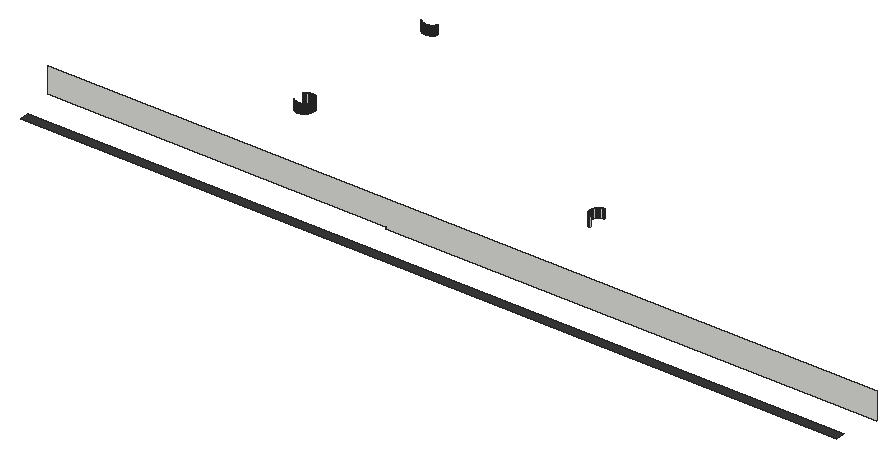
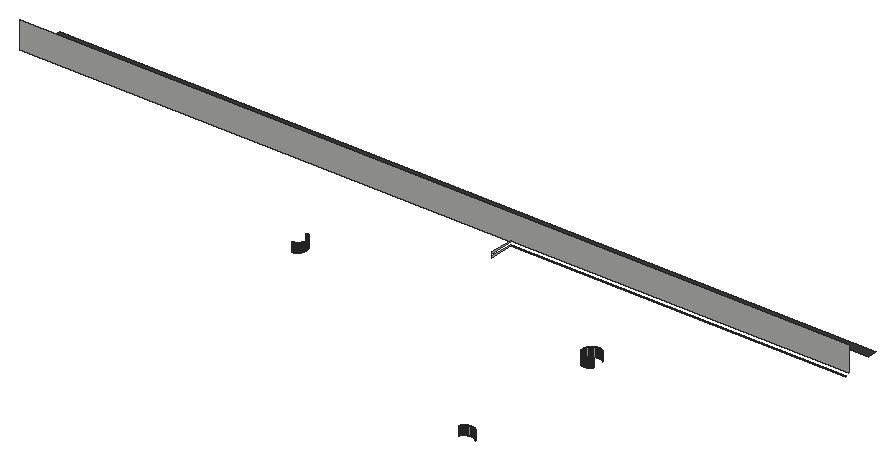
# SketchUp Ruby script. Lengths in inches.
U = 1.inch
M = Sketchup.active_model
def pt(a) = Geom::Point3d.new(a.map { |v| v * U })
def face(e, loops, mat)
  f = e.add_face(loops[0].map { |a| pt(a) })
  loops[1..].each { |l| e.add_face(l.map { |a| pt(a) }).erase! }
  f.material = f.back_material = mat if mat
  f
end
# faces: each face lists its corners as indices into pts; further lists are holes
def faces(e, pts, list, mat = nil) = list.each { |f| face(e, (f[0].is_a?(Array) ? f : [f]).map { |l| l.map { |i| pts[i] } }, mat) }
# xy, xz, yz: faces in a plane at the given z, y or x. An outline is a flat list of corners, or four numbers for a rectangle; further outlines are holes
def ring(l) = l.size == 4 ? [[l[0], l[1]], [l[2], l[1]], [l[2], l[3]], [l[0], l[3]]] : l.each_slice(2).to_a
def flat(e, list, mat, &to3) = list.each { |f| face(e, (f[0].is_a?(Array) ? f : [f]).map { |l| ring(l).map { |u, v| to3.(u, v) } }, mat) }
def xy(e, z, list, mat = nil) = flat(e, list, mat) { |x, y| [x, y, z] }
def xz(e, y, list, mat = nil) = flat(e, list, mat) { |x, z| [x, y, z] }
def yz(e, x, list, mat = nil) = flat(e, list, mat) { |y, z| [x, y, z] }
def lines(e, pts, list) = list.each { |a, b| e.add_line(pt(pts[a]), pt(pts[b])) }
# prism: a flat outline (further loops are holes) pulled along v
def prism(e, loops, v, mat = nil)
  f = face(e, loops, mat); d = Geom::Vector3d.new(v.map { |x| x * U })
  f.pushpull(f.normal.samedirection?(d) ? d.length : -d.length)
end
def box(e, o, s, mat = nil) = prism(e, [[o, [o[0] + s[0], o[1], o[2]], [o[0] + s[0], o[1] + s[1], o[2]], [o[0], o[1] + s[1], o[2]]]], [0, 0, s[2]], mat)
def at(x, y, z, deg = 0) = Geom::Transformation.translation(pt([x, y, z])) * Geom::Transformation.rotation(ORIGIN, Z_AXIS, deg.degrees)
def axes(o, x, y, z) = Geom::Transformation.new([*x, 0, *y, 0, *z, 0, *pt(o).to_a, 1])
def part(name) = M.definitions.add(name)
# library, detail: a bought-in or finely detailed component or shape, given as its bounding box
def library(name, o, s) = part(name).tap { |d| box(d.entities, o, s) }
def detail(e, o, s) = box(e.add_group.entities, o, s)
def put(e, d, t, mat = nil) = e.add_instance(d, t).tap { |i| i.material = mat if mat }
def group(e, t, mat = nil) = e.add_group.tap { |g| g.transformation = t; g.material = mat if mat }.entities
root = M.entities
M.materials.add("1496 AP 8293 CARBON COPY").color = [58, 58, 58]
xy(root,129,[[46,71,321,74]],"1496 AP 8293 CARBON COPY")
xz(root,85,[[158,129,323,129,323,138,44,138,44,129.5,158,129.5]])
xz(root,86.5,[[44,129,156.5,129.5]])
xz(root,119,[[100.84,129,100.92,132],[100.92,129,101,132],[101,129,101.08,132],[101.08,129,101.16,132]])
xz(root,125,[[100.84,129,100.92,132],[100.92,129,101,132],[101,129,101.08,132],[101.08,129,101.16,132]])
xz(root,172.75,[[100.84,129,100.92,132],[100.92,129,101,132],[101,129,101.08,132],[101.08,129,101.16,132]])
yz(root,104,[[121.84,129,121.92,132],[121.92,129,122,132],[122,129,122.08,132],[122.08,129,122.16,132]])
yz(root,156.5,[[86.5,129,94.5,129.5]])
yz(root,158,[[85,129,93,129.5]])
yz(root,197,[[121.84,129,121.92,132],[121.92,129,122,132],[122,129,122.08,132],[122.08,129,122.16,132]])
p = [[100.53,119.04,129],[100.45,119.05,129],[100.45,119.05,132],[100.53,119.04,132],[100.61,119.03,129],[100.61,119.03,132],
  [100.6875,119.02,129],[100.6875,119.02,132],[100.76,119.01,129],[100.76,119.01,132],[100.84,119,129],[100.84,119,132],
  [101.24,119.01,129],[101.16,119,129],[101.16,119,132],[101.24,119.01,132],[101.3125,119.02,129],[101.3125,119.02,132],
  [101.39,119.03,129],[101.39,119.03,132],[101.47,119.04,129],[101.47,119.04,132],[101.55,119.05,129],[101.55,119.05,132],
  [199.53,119.04,129],[199.45,119.05,129],[199.45,119.05,132],[199.53,119.04,132],[100.07,119.15,129],[100,119.17,129],
  [100,119.17,132],[100.07,119.15,132],[100.15,119.125,129],[100.15,119.125,132],[100.22,119.1,129],[100.22,119.1,132],
  [100.3,119.08,129],[100.3,119.08,132],[100.375,119.07,129],[100.375,119.07,132],[101.625,119.07,129],[101.625,119.07,132],
  [101.7,119.08,129],[101.7,119.08,132],[101.78,119.1,129],[101.78,119.1,132],[101.85,119.125,129],[101.85,119.125,132],
  [101.93,119.15,129],[101.93,119.15,132],[102,119.17,129],[102,119.17,132],[199.07,119.15,129],[199,119.17,129],
  [199,119.17,132],[199.07,119.15,132],[199.15,119.125,129],[199.15,119.125,132],[199.22,119.1,129],[199.22,119.1,132],
  [199.3,119.08,129],[199.3,119.08,132],[199.375,119.07,129],[199.375,119.07,132],[99.85,119.23,129],[99.78,119.26,129],
  [99.78,119.26,132],[99.85,119.23,132],[99.92,119.2,129],[99.92,119.2,132],[102.08,119.2,129],[102.08,119.2,132],
  [102.15,119.23,129],[102.15,119.23,132],[102.22,119.26,129],[102.22,119.26,132],[198.85,119.23,129],[198.78,119.26,129],
  [198.78,119.26,132],[198.85,119.23,132],[198.92,119.2,129],[198.92,119.2,132],[99.64,119.33,129],[99.57,119.36,129],
  [99.57,119.36,132],[99.64,119.33,132],[99.71,119.29,129],[99.71,119.29,132],[102.29,119.29,129],[102.29,119.29,132],
  [102.36,119.33,129],[102.36,119.33,132],[102.43,119.36,129],[102.43,119.36,132],[198.64,119.33,129],[198.57,119.36,129],
  [198.57,119.36,132],[198.64,119.33,132],[198.71,119.29,129],[198.71,119.29,132],[99.43,119.44,129],[99.37,119.48,129],
  [99.37,119.48,132],[99.43,119.44,132],[99.5,119.4,129],[99.5,119.4,132],[102.5,119.4,129],[102.5,119.4,132],
  [102.57,119.44,129],[102.57,119.44,132],[102.63,119.48,129],[102.63,119.48,132],[198.43,119.44,129],[198.37,119.48,129],
  [198.37,119.48,132],[198.43,119.44,132],[198.5,119.4,129],[198.5,119.4,132],[99.3,119.53,129],[99.24,119.57,129],
  [99.24,119.57,132],[99.3,119.53,132],[102.7,119.53,129],[102.7,119.53,132],[102.76,119.57,129],[102.76,119.57,132],
  [198.3,119.53,129],[198.24,119.57,129],[198.24,119.57,132],[198.3,119.53,132],[99.17,119.62,129],[99.11,119.67,129],
  [99.11,119.67,132],[99.17,119.62,132],[102.83,119.62,129],[102.83,119.62,132],[102.89,119.67,129],[102.89,119.67,132],
  [198.17,119.62,129],[198.11,119.67,129],[198.11,119.67,132],[198.17,119.62,132],[99.05,119.72,129],[98.99,119.77,129],
  [98.99,119.77,132],[99.05,119.72,132],[102.95,119.72,129],[102.95,119.72,132],[103.01,119.77,129],[103.01,119.77,132],
  [198.05,119.72,129],[197.99,119.77,129],[197.99,119.77,132],[198.05,119.72,132],[98.93,119.82,129],[98.88,119.88,129],
  [98.88,119.88,132],[98.93,119.82,132],[103.07,119.82,129],[103.07,119.82,132],[103.12,119.88,129],[103.12,119.88,132],
  [197.93,119.82,129],[197.88,119.88,129],[197.88,119.88,132],[197.93,119.82,132],[98.82,119.93,129],[98.77,119.99,129],
  [98.77,119.99,132],[98.82,119.93,132],[103.18,119.93,129],[103.18,119.93,132],[103.23,119.99,129],[103.23,119.99,132],
  [197.82,119.93,129],[197.77,119.99,129],[197.77,119.99,132],[197.82,119.93,132],[98.72,120.05,129],[98.72,120.05,132],
  [103.28,120.05,129],[103.28,120.05,132],[197.72,120.05,129],[197.72,120.05,132],[103.33,120.11,129],[103.33,120.11,132],
  [103.38,120.17,129],[103.38,120.17,132],[197.67,120.11,129],[197.62,120.17,129],[197.62,120.17,132],[197.67,120.11,132],
  [103.43,120.24,129],[103.43,120.24,132],[103.47,120.3,129],[103.47,120.3,132],[197.57,120.24,129],[197.53,120.3,129],
  [197.53,120.3,132],[197.57,120.24,132],[103.52,120.37,129],[103.52,120.37,132],[197.48,120.37,129],[197.48,120.37,132],
  [103.56,120.43,129],[103.56,120.43,132],[103.6,120.5,129],[103.6,120.5,132],[197.44,120.43,129],[197.4,120.5,129],
  [197.4,120.5,132],[197.44,120.43,132],[103.64,120.57,129],[103.64,120.57,132],[197.36,120.57,129],[197.36,120.57,132],
  [103.67,120.64,129],[103.67,120.64,132],[103.71,120.71,129],[103.71,120.71,132],[197.33,120.64,129],[197.29,120.71,129],
  [197.29,120.71,132],[197.33,120.64,132],[103.74,120.78,129],[103.74,120.78,132],[197.26,120.78,129],[197.26,120.78,132],
  [103.77,120.85,129],[103.77,120.85,132],[197.23,120.85,129],[197.23,120.85,132],[103.8,120.92,129],[103.8,120.92,132],
  [103.83,121,129],[103.83,121,132],[197.2,120.92,129],[197.17,121,129],[197.17,121,132],[197.2,120.92,132],
  [103.85,121.07,129],[103.85,121.07,132],[197.15,121.07,129],[197.15,121.07,132],[103.875,121.15,129],[103.875,121.15,132],
  [103.9,121.22,129],[103.9,121.22,132],[197.125,121.15,129],[197.1,121.22,129],[197.1,121.22,132],[197.125,121.15,132],
  [103.92,121.3,129],[103.92,121.3,132],[197.08,121.3,129],[197.08,121.3,132],[103.93,121.375,129],[103.93,121.375,132],
  [197.07,121.375,129],[197.07,121.375,132],[103.95,121.45,129],[103.95,121.45,132],[197.05,121.45,129],[197.05,121.45,132],
  [103.96,121.53,129],[103.96,121.53,132],[103.97,121.61,129],[103.97,121.61,132],[197.04,121.53,129],[197.03,121.61,129],
  [197.03,121.61,132],[197.04,121.53,132],[103.98,121.6875,129],[103.98,121.6875,132],[197.02,121.6875,129],[197.02,121.6875,132],
  [103.99,121.76,129],[103.99,121.76,132],[197.01,121.76,129],[197.01,121.76,132],[104,121.84,129],[104,121.84,132],
  [197,121.84,129],[197,121.84,132],[103.98,122.3125,129],[103.99,122.24,129],[103.99,122.24,132],[103.98,122.3125,132],
  [104,122.16,129],[104,122.16,132],[197,122.16,129],[197.01,122.24,129],[197.01,122.24,132],[197,122.16,132],
  [197.02,122.3125,129],[197.02,122.3125,132],[103.97,122.39,129],[103.97,122.39,132],[197.03,122.39,129],[197.03,122.39,132],
  [103.96,122.47,129],[103.96,122.47,132],[197.04,122.47,129],[197.04,122.47,132],[103.93,122.625,129],[103.95,122.55,129],
  [103.95,122.55,132],[103.93,122.625,132],[197.05,122.55,129],[197.05,122.55,132],[197.07,122.625,129],[197.07,122.625,132],
  [103.92,122.7,129],[103.92,122.7,132],[197.08,122.7,129],[197.08,122.7,132],[103.9,122.78,129],[103.9,122.78,132],
  [197.1,122.78,129],[197.1,122.78,132],[103.875,122.85,129],[103.875,122.85,132],[197.125,122.85,129],[197.125,122.85,132],
  [103.83,123,129],[103.85,122.93,129],[103.85,122.93,132],[103.83,123,132],[197.15,122.93,129],[197.15,122.93,132],
  [197.17,123,129],[197.17,123,132],[103.8,123.08,129],[103.8,123.08,132],[197.2,123.08,129],[197.2,123.08,132],
  [103.74,123.22,129],[103.77,123.15,129],[103.77,123.15,132],[103.74,123.22,132],[197.23,123.15,129],[197.23,123.15,132],
  [197.26,123.22,129],[197.26,123.22,132],[103.71,123.29,129],[103.71,123.29,132],[197.29,123.29,129],[197.29,123.29,132],
  [103.67,123.36,129],[103.67,123.36,132],[197.33,123.36,129],[197.33,123.36,132],[103.6,123.5,129],[103.64,123.43,129],
  [103.64,123.43,132],[103.6,123.5,132],[197.36,123.43,129],[197.36,123.43,132],[197.4,123.5,129],[197.4,123.5,132],
  [103.56,123.57,129],[103.56,123.57,132],[197.44,123.57,129],[197.44,123.57,132],[103.47,123.7,129],[103.52,123.63,129],
  [103.52,123.63,132],[103.47,123.7,132],[197.48,123.63,129],[197.48,123.63,132],[197.53,123.7,129],[197.53,123.7,132],
  [103.43,123.76,129],[103.43,123.76,132],[197.57,123.76,129],[197.57,123.76,132],[103.33,123.89,129],[103.38,123.83,129],
  [103.38,123.83,132],[103.33,123.89,132],[197.62,123.83,129],[197.62,123.83,132],[197.67,123.89,129],[197.67,123.89,132],
  [98.72,123.95,129],[98.77,124.01,129],[98.77,124.01,132],[98.72,123.95,132],[103.23,124.01,129],[103.28,123.95,129],
  [103.28,123.95,132],[103.23,124.01,132],[197.72,123.95,129],[197.72,123.95,132],[197.77,124.01,129],[197.77,124.01,132],
  [98.82,124.07,129],[98.82,124.07,132],[103.18,124.07,129],[103.18,124.07,132],[197.82,124.07,129],[197.82,124.07,132],
  [98.88,124.12,129],[98.88,124.12,132],[98.93,124.18,129],[98.93,124.18,132],[103.07,124.18,129],[103.12,124.12,129],
  [103.12,124.12,132],[103.07,124.18,132],[197.88,124.12,129],[197.88,124.12,132],[197.93,124.18,129],[197.93,124.18,132],
  [98.99,124.23,129],[98.99,124.23,132],[99.05,124.28,129],[99.05,124.28,132],[102.95,124.28,129],[103.01,124.23,129],
  [103.01,124.23,132],[102.95,124.28,132],[197.99,124.23,129],[197.99,124.23,132],[198.05,124.28,129],[198.05,124.28,132],
  [99.11,124.33,129],[99.11,124.33,132],[99.17,124.38,129],[99.17,124.38,132],[102.83,124.38,129],[102.89,124.33,129],
  [102.89,124.33,132],[102.83,124.38,132],[198.11,124.33,129],[198.11,124.33,132],[198.17,124.38,129],[198.17,124.38,132],
  [99.24,124.43,129],[99.24,124.43,132],[99.3,124.47,129],[99.3,124.47,132],[102.7,124.47,129],[102.76,124.43,129],
  [102.76,124.43,132],[102.7,124.47,132],[198.24,124.43,129],[198.24,124.43,132],[198.3,124.47,129],[198.3,124.47,132],
  [99.37,124.52,129],[99.37,124.52,132],[99.43,124.56,129],[99.43,124.56,132],[102.57,124.56,129],[102.63,124.52,129],
  [102.63,124.52,132],[102.57,124.56,132],[198.37,124.52,129],[198.37,124.52,132],[198.43,124.56,129],[198.43,124.56,132],
  [99.5,124.6,129],[99.5,124.6,132],[99.57,124.64,129],[99.57,124.64,132],[99.64,124.67,129],[99.64,124.67,132],
  [102.36,124.67,129],[102.43,124.64,129],[102.43,124.64,132],[102.36,124.67,132],[102.5,124.6,129],[102.5,124.6,132],
  [198.5,124.6,129],[198.5,124.6,132],[198.57,124.64,129],[198.57,124.64,132],[198.64,124.67,129],[198.64,124.67,132],
  [99.71,124.71,129],[99.71,124.71,132],[99.78,124.74,129],[99.78,124.74,132],[99.85,124.77,129],[99.85,124.77,132],
  [102.15,124.77,129],[102.22,124.74,129],[102.22,124.74,132],[102.15,124.77,132],[102.29,124.71,129],[102.29,124.71,132],
  [198.71,124.71,129],[198.71,124.71,132],[198.78,124.74,129],[198.78,124.74,132],[198.85,124.77,129],[198.85,124.77,132],
  [99.92,124.8,129],[99.92,124.8,132],[100,124.83,129],[100,124.83,132],[100.07,124.85,129],[100.07,124.85,132],
  [101.93,124.85,129],[102,124.83,129],[102,124.83,132],[101.93,124.85,132],[102.08,124.8,129],[102.08,124.8,132],
  [198.92,124.8,129],[198.92,124.8,132],[199,124.83,129],[199,124.83,132],[199.07,124.85,129],[199.07,124.85,132],
  [100.15,124.875,129],[100.15,124.875,132],[100.22,124.9,129],[100.22,124.9,132],[100.3,124.92,129],[100.3,124.92,132],
  [100.375,124.93,129],[100.375,124.93,132],[100.45,124.95,129],[100.45,124.95,132],[100.53,124.96,129],[100.53,124.96,132],
  [101.47,124.96,129],[101.55,124.95,129],[101.55,124.95,132],[101.47,124.96,132],[101.625,124.93,129],[101.625,124.93,132],
  [101.7,124.92,129],[101.7,124.92,132],[101.78,124.9,129],[101.78,124.9,132],[101.85,124.875,129],[101.85,124.875,132],
  [199.15,124.875,129],[199.15,124.875,132],[199.22,124.9,129],[199.22,124.9,132],[199.3,124.92,129],[199.3,124.92,132],
  [199.375,124.93,129],[199.375,124.93,132],[199.45,124.95,129],[199.45,124.95,132],[199.53,124.96,129],[199.53,124.96,132],
  [100.61,124.97,129],[100.61,124.97,132],[100.6875,124.98,129],[100.6875,124.98,132],[100.76,124.99,129],[100.76,124.99,132],
  [100.84,125,129],[100.84,125,132],[101.16,125,129],[101.24,124.99,129],[101.24,124.99,132],[101.16,125,132],
  [101.3125,124.98,129],[101.3125,124.98,132],[101.39,124.97,129],[101.39,124.97,132],[199.61,124.97,129],[199.61,124.97,132],
  [100.3,172.83,129],[100.22,172.85,129],[100.22,172.85,132],[100.3,172.83,132],[100.375,172.82,129],[100.375,172.82,132],
  [100.45,172.8,129],[100.45,172.8,132],[100.53,172.79,129],[100.53,172.79,132],[100.61,172.78,129],[100.61,172.78,132],
  [100.6875,172.77,129],[100.6875,172.77,132],[100.76,172.76,129],[100.76,172.76,132],[100.84,172.75,129],[100.84,172.75,132],
  [101.24,172.76,129],[101.16,172.75,129],[101.16,172.75,132],[101.24,172.76,132],[101.3125,172.77,129],[101.3125,172.77,132],
  [101.39,172.78,129],[101.39,172.78,132],[101.47,172.79,129],[101.47,172.79,132],[101.55,172.8,129],[101.55,172.8,132],
  [101.625,172.82,129],[101.625,172.82,132],[101.7,172.83,129],[101.7,172.83,132],[101.78,172.85,129],[101.78,172.85,132],
  [99.92,172.95,129],[99.85,172.98,129],[99.85,172.98,132],[99.92,172.95,132],[100,172.92,129],[100,172.92,132],
  [100.07,172.9,129],[100.07,172.9,132],[100.15,172.875,129],[100.15,172.875,132],[101.85,172.875,129],[101.85,172.875,132],
  [101.93,172.9,129],[101.93,172.9,132],[102,172.92,129],[102,172.92,132],[102.08,172.95,129],[102.08,172.95,132],
  [102.15,172.98,129],[102.15,172.98,132],[99.71,173.04,129],[99.64,173.08,129],[99.64,173.08,132],[99.71,173.04,132],
  [99.78,173.01,129],[99.78,173.01,132],[102.22,173.01,129],[102.22,173.01,132],[102.29,173.04,129],[102.29,173.04,132],
  [102.36,173.08,129],[102.36,173.08,132],[99.57,173.11,129],[99.5,173.15,129],[99.5,173.15,132],[99.57,173.11,132],
  [102.43,173.11,129],[102.43,173.11,132],[102.5,173.15,129],[102.5,173.15,132],[99.37,173.23,129],[99.3,173.28,129],
  [99.3,173.28,132],[99.37,173.23,132],[99.43,173.19,129],[99.43,173.19,132],[102.57,173.19,129],[102.57,173.19,132],
  [102.63,173.23,129],[102.63,173.23,132],[102.7,173.28,129],[102.7,173.28,132],[99.24,173.32,129],[99.17,173.37,129],
  [99.17,173.37,132],[99.24,173.32,132],[102.76,173.32,129],[102.76,173.32,132],[102.83,173.37,129],[102.83,173.37,132],
  [99.11,173.42,129],[99.05,173.47,129],[99.05,173.47,132],[99.11,173.42,132],[102.89,173.42,129],[102.89,173.42,132],
  [102.95,173.47,129],[102.95,173.47,132],[98.99,173.52,129],[98.93,173.57,129],[98.93,173.57,132],[98.99,173.52,132],
  [103.01,173.52,129],[103.01,173.52,132],[103.07,173.57,129],[103.07,173.57,132],[98.88,173.63,129],[98.82,173.68,129],
  [98.82,173.68,132],[98.88,173.63,132],[103.12,173.63,129],[103.12,173.63,132],[103.18,173.68,129],[103.18,173.68,132],
  [98.77,173.74,129],[98.72,173.8,129],[98.72,173.8,132],[98.77,173.74,132],[103.23,173.74,129],[103.23,173.74,132],
  [103.28,173.8,129],[103.28,173.8,132],[98.67,173.86,129],[98.67,173.86,132],[103.33,173.86,129],[103.33,173.86,132],
  [103.38,173.92,129],[103.38,173.92,132],[103.43,173.99,129],[103.43,173.99,132],[103.47,174.05,129],[103.47,174.05,132],
  [103.52,174.12,129],[103.52,174.12,132],[103.56,174.18,129],[103.56,174.18,132],[103.6,174.25,129],[103.6,174.25,132],
  [103.64,174.32,129],[103.64,174.32,132],[103.67,174.39,129],[103.67,174.39,132],[103.71,174.46,129],[103.71,174.46,132],
  [103.74,174.53,129],[103.74,174.53,132],[103.77,174.6,129],[103.77,174.6,132]]
faces(root,p,[[0,1,2,3],[4,0,3,5],[6,4,5,7],[8,6,7,9],[10,8,9,11],[12,13,14,15],[16,12,15,17],[18,16,17,19],
  [20,18,19,21],[22,20,21,23],[24,25,26,27],[28,29,30,31],[32,28,31,33],[34,32,33,35],[36,34,35,37],[38,36,37,39],
  [1,38,39,2],[40,22,23,41],[42,40,41,43],[44,42,43,45],[46,44,45,47],[48,46,47,49],[50,48,49,51],[52,53,54,55],
  [56,52,55,57],[58,56,57,59],[60,58,59,61],[62,60,61,63],[25,62,63,26],[64,65,66,67],[68,64,67,69],[29,68,69,30],
  [70,50,51,71],[72,70,71,73],[74,72,73,75],[76,77,78,79],[80,76,79,81],[53,80,81,54],[82,83,84,85],[86,82,85,87],
  [65,86,87,66],[88,74,75,89],[90,88,89,91],[92,90,91,93],[94,95,96,97],[98,94,97,99],[77,98,99,78],[100,101,102,103],
  [104,100,103,105],[83,104,105,84],[106,92,93,107],[108,106,107,109],[110,108,109,111],[112,113,114,115],[116,112,115,117],[95,116,117,96],
  [118,119,120,121],[101,118,121,102],[122,110,111,123],[124,122,123,125],[126,127,128,129],[113,126,129,114],[130,131,132,133],[119,130,133,120],
  [134,124,125,135],[136,134,135,137],[138,139,140,141],[127,138,141,128],[142,143,144,145],[131,142,145,132],[146,136,137,147],[148,146,147,149],
  [150,151,152,153],[139,150,153,140],[154,155,156,157],[143,154,157,144],[158,148,149,159],[160,158,159,161],[162,163,164,165],[151,162,165,152],
  [166,167,168,169],[155,166,169,156],[170,160,161,171],[172,170,171,173],[174,175,176,177],[163,174,177,164],[167,178,179,168],[180,172,173,181],
  [175,182,183,176],[184,180,181,185],[186,184,185,187],[188,189,190,191],[182,188,191,183],[192,186,187,193],[194,192,193,195],[196,197,198,199],
  [189,196,199,190],[200,194,195,201],[197,202,203,198],[204,200,201,205],[206,204,205,207],[208,209,210,211],[202,208,211,203],[212,206,207,213],
  [209,214,215,210],[216,212,213,217],[218,216,217,219],[220,221,222,223],[214,220,223,215],[224,218,219,225],[221,226,227,222],[228,224,225,229],
  [226,230,231,227],[232,228,229,233],[234,232,233,235],[236,237,238,239],[230,236,239,231],[240,234,235,241],[237,242,243,238],[244,240,241,245],
  [246,244,245,247],[248,249,250,251],[242,248,251,243],[252,246,247,253],[249,254,255,250],[256,252,253,257],[254,258,259,255],[260,256,257,261],
  [258,262,263,259],[264,260,261,265],[266,264,265,267],[268,269,270,271],[262,268,271,263],[272,266,267,273],[269,274,275,270],[276,272,273,277],
  [274,278,279,275],[280,276,277,281],[278,282,283,279],[284,285,286,287],[285,288,289,286],[290,291,292,293],[291,294,295,292],[296,284,287,297],
  [294,298,299,295],[300,296,297,301],[298,302,303,299],[304,305,306,307],[305,300,301,306],[302,308,309,303],[308,310,311,309],[312,304,307,313],
  [310,314,315,311],[316,312,313,317],[314,318,319,315],[320,316,317,321],[318,322,323,319],[324,325,326,327],[325,320,321,326],[322,328,329,323],
  [328,330,331,329],[332,324,327,333],[330,334,335,331],[336,337,338,339],[337,332,333,338],[334,340,341,335],[340,342,343,341],[344,336,339,345],
  [342,346,347,343],[348,344,345,349],[346,350,351,347],[352,353,354,355],[353,348,349,354],[350,356,357,351],[356,358,359,357],[360,352,355,361],
  [358,362,363,359],[364,365,366,367],[365,360,361,366],[362,368,369,363],[368,370,371,369],[372,364,367,373],[370,374,375,371],[376,377,378,379],
  [377,372,373,378],[374,380,381,375],[380,382,383,381],[384,385,386,387],[388,389,390,391],[389,376,379,390],[382,392,393,383],[392,394,395,393],
  [385,396,397,386],[398,388,391,399],[394,400,401,395],[396,402,403,397],[402,404,405,403],[406,407,408,409],[407,398,399,408],[400,410,411,401],
  [410,412,413,411],[404,414,415,405],[414,416,417,415],[418,419,420,421],[419,406,409,420],[412,422,423,413],[422,424,425,423],[416,426,427,417],
  [426,428,429,427],[430,431,432,433],[431,418,421,432],[424,434,435,425],[434,436,437,435],[428,438,439,429],[438,440,441,439],[442,443,444,445],
  [443,430,433,444],[436,446,447,437],[446,448,449,447],[440,450,451,441],[450,452,453,451],[454,455,456,457],[455,442,445,456],[448,458,459,449],
  [458,460,461,459],[452,462,463,453],[462,464,465,463],[464,466,467,465],[468,469,470,471],[469,472,473,470],[472,454,457,473],[460,474,475,461],
  [474,476,477,475],[476,478,479,477],[466,480,481,467],[480,482,483,481],[482,484,485,483],[486,487,488,489],[487,490,491,488],[490,468,471,491],
  [478,492,493,479],[492,494,495,493],[494,496,497,495],[484,498,499,485],[498,500,501,499],[500,502,503,501],[504,505,506,507],[505,508,509,506],
  [508,486,489,509],[496,510,511,497],[510,512,513,511],[512,514,515,513],[502,516,517,503],[516,518,519,517],[518,520,521,519],[520,522,523,521],
  [522,524,525,523],[524,526,527,525],[528,529,530,531],[529,532,533,530],[532,534,535,533],[534,536,537,535],[536,538,539,537],[538,504,507,539],
  [514,540,541,515],[540,542,543,541],[542,544,545,543],[544,546,547,545],[546,548,549,547],[548,550,551,549],[526,552,553,527],[552,554,555,553],
  [554,556,557,555],[556,558,559,557],[560,561,562,563],[561,564,565,562],[564,566,567,565],[566,528,531,567],[550,568,569,551],[570,571,572,573],
  [574,570,573,575],[576,574,575,577],[578,576,577,579],[580,578,579,581],[582,580,581,583],[584,582,583,585],[586,584,585,587],[588,589,590,591],
  [592,588,591,593],[594,592,593,595],[596,594,595,597],[598,596,597,599],[600,598,599,601],[602,600,601,603],[604,602,603,605],[606,607,608,609],
  [610,606,609,611],[612,610,611,613],[614,612,613,615],[571,614,615,572],[616,604,605,617],[618,616,617,619],[620,618,619,621],[622,620,621,623],
  [624,622,623,625],[626,627,628,629],[630,626,629,631],[607,630,631,608],[632,624,625,633],[634,632,633,635],[636,634,635,637],[638,639,640,641],
  [627,638,641,628],[642,636,637,643],[644,642,643,645],[646,647,648,649],[650,646,649,651],[639,650,651,640],[652,644,645,653],[654,652,653,655],
  [656,654,655,657],[658,659,660,661],[647,658,661,648],[662,656,657,663],[664,662,663,665],[666,667,668,669],[659,666,669,660],[670,664,665,671],
  [672,670,671,673],[674,675,676,677],[667,674,677,668],[678,672,673,679],[680,678,679,681],[682,683,684,685],[675,682,685,676],[686,680,681,687],
  [688,686,687,689],[690,691,692,693],[683,690,693,684],[694,688,689,695],[696,694,695,697],[691,698,699,692],[700,696,697,701],[702,700,701,703],
  [704,702,703,705],[706,704,705,707],[708,706,707,709],[710,708,709,711],[712,710,711,713],[714,712,713,715],[716,714,715,717],[718,716,717,719],
  [720,718,719,721],[722,720,721,723]])
